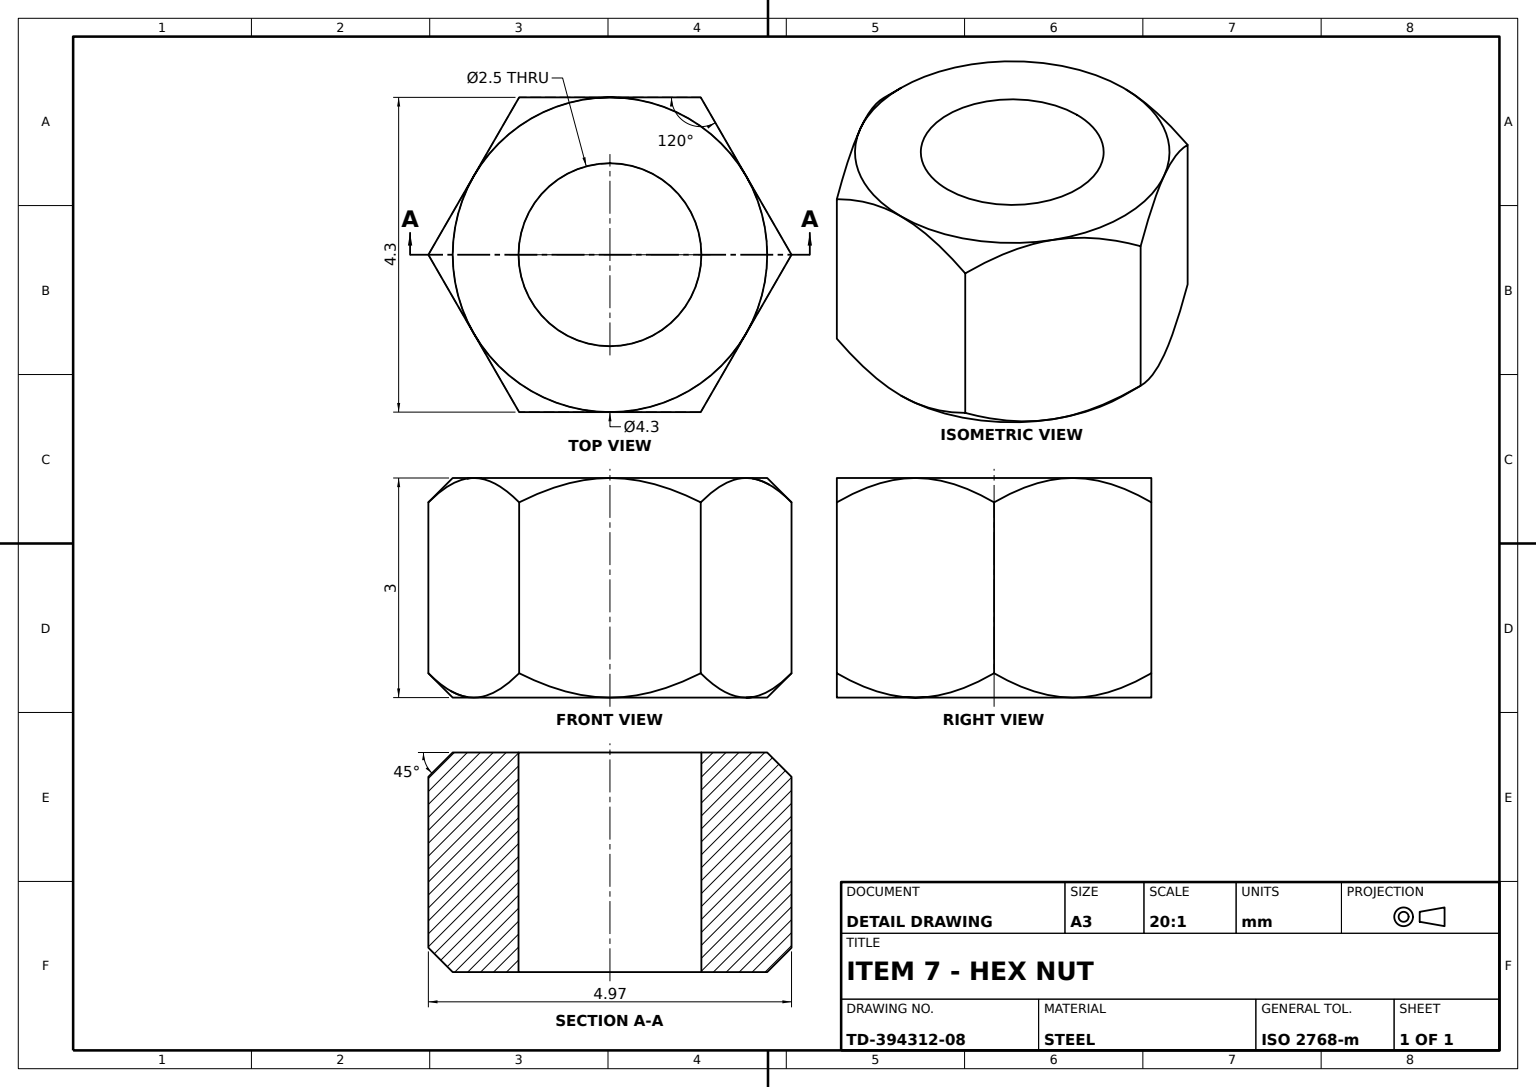
ISO-10303-21;
HEADER;
FILE_DESCRIPTION((''),'2;1');
FILE_NAME('','',(''),(''),'','','');
FILE_SCHEMA(('AUTOMOTIVE_DESIGN'));
ENDSEC;
DATA;
#1=APPLICATION_CONTEXT('');
#2=PRODUCT_CONTEXT('',#1,'mechanical');
#3=PRODUCT('','','',(#2));
#4=PRODUCT_DEFINITION_FORMATION('','',#3);
#5=PRODUCT_DEFINITION_CONTEXT('',#1,'design');
#6=PRODUCT_DEFINITION('','',#4,#5);
#7=PRODUCT_DEFINITION_SHAPE('','',#6);
#8=(LENGTH_UNIT()NAMED_UNIT(*)SI_UNIT(.MILLI.,.METRE.));
#9=(NAMED_UNIT(*)PLANE_ANGLE_UNIT()SI_UNIT($,.RADIAN.));
#10=(NAMED_UNIT(*)SI_UNIT($,.STERADIAN.)SOLID_ANGLE_UNIT());
#11=UNCERTAINTY_MEASURE_WITH_UNIT(LENGTH_MEASURE(1.E-05),#8,'distance_accuracy_value','');
#12=(GEOMETRIC_REPRESENTATION_CONTEXT(3)GLOBAL_UNCERTAINTY_ASSIGNED_CONTEXT((#11))GLOBAL_UNIT_ASSIGNED_CONTEXT((#8,#9,#10))REPRESENTATION_CONTEXT('',''));
#13=CARTESIAN_POINT('',(-1.861955,3.,-1.075));
#14=VERTEX_POINT('',#13);
#15=CARTESIAN_POINT('',(-2.482606,2.667394,0.));
#16=VERTEX_POINT('',#15);
#17=CARTESIAN_POINT('',(-1.969911,3.,-0.888014));
#18=CARTESIAN_POINT('',(-2.076031,2.966986,-0.704208));
#19=CARTESIAN_POINT('',(-2.285328,2.847997,-0.341695));
#20=CARTESIAN_POINT('',(-2.385392,2.764608,-0.16838));
#21=B_SPLINE_CURVE_WITH_KNOTS('',3,(#13,#17,#18,#19,#20,#15),.UNSPECIFIED.,.F.,.F.,(4,2,4),(0.001286977,0.00192583,0.002564683),.UNSPECIFIED.);
#22=EDGE_CURVE('',#14,#16,#21,.T.);
#23=ORIENTED_EDGE('',*,*,#22,.T.);
#24=CARTESIAN_POINT('',(-1.861955,3.,1.075));
#25=VERTEX_POINT('',#24);
#26=CARTESIAN_POINT('',(-2.38528,2.76472,0.168574));
#27=CARTESIAN_POINT('',(-2.28575,2.847423,0.340964));
#28=CARTESIAN_POINT('',(-2.131089,2.935848,0.608845));
#29=CARTESIAN_POINT('',(-2.078631,2.959321,0.699705));
#30=CARTESIAN_POINT('',(-1.971486,2.991467,0.885286));
#31=CARTESIAN_POINT('',(-1.916314,3.,0.980847));
#32=B_SPLINE_CURVE_WITH_KNOTS('',3,(#15,#26,#27,#28,#29,#30,#31,#24),.UNSPECIFIED.,.F.,.F.,(4,2,2,4),(0.000000254,0.000643616,0.000965296,0.001286977),.UNSPECIFIED.);
#33=EDGE_CURVE('',#16,#25,#32,.T.);
#34=ORIENTED_EDGE('',*,*,#33,.T.);
#35=CARTESIAN_POINT('',(0.,3.,0.));
#36=DIRECTION('',(0.,1.,0.));
#37=DIRECTION('',(0.,0.,1.));
#38=AXIS2_PLACEMENT_3D('',#35,#36,#37);
#39=CIRCLE('',#38,2.15);
#40=EDGE_CURVE('',#14,#25,#39,.T.);
#41=ORIENTED_EDGE('',*,*,#40,.F.);
#42=EDGE_LOOP('',(#23,#34,#41));
#43=FACE_OUTER_BOUND('',#42,.T.);
#44=DIRECTION('',(0.,-1.,0.));
#45=AXIS2_PLACEMENT_3D('',#35,#44,#37);
#46=CONICAL_SURFACE('',#45,2.15,0.785398163);
#47=ADVANCED_FACE('',(#43),#46,.T.);
#48=CARTESIAN_POINT('',(0.,0.,-2.15));
#49=VERTEX_POINT('',#48);
#50=CARTESIAN_POINT('',(1.241303,0.332606,-2.15));
#51=VERTEX_POINT('',#50);
#52=CARTESIAN_POINT('',(0.108245,0.,-2.15));
#53=CARTESIAN_POINT('',(0.217598,0.008403,-2.15));
#54=CARTESIAN_POINT('',(0.431131,0.040258,-2.15));
#55=CARTESIAN_POINT('',(0.536253,0.063635,-2.15));
#56=CARTESIAN_POINT('',(0.847499,0.152434,-2.15));
#57=CARTESIAN_POINT('',(1.049442,0.236676,-2.15));
#58=B_SPLINE_CURVE_WITH_KNOTS('',3,(#48,#52,#53,#54,#55,#56,#57,#50),.UNSPECIFIED.,.F.,.F.,(4,2,2,4),(0.005941609,0.00626575,0.006589892,0.007238175),.UNSPECIFIED.);
#59=EDGE_CURVE('',#49,#51,#58,.T.);
#60=ORIENTED_EDGE('',*,*,#59,.F.);
#61=CARTESIAN_POINT('',(-1.241303,0.332606,-2.15));
#62=VERTEX_POINT('',#61);
#63=CARTESIAN_POINT('',(-1.048003,0.235956,-2.15));
#64=CARTESIAN_POINT('',(-0.848605,0.152667,-2.15));
#65=CARTESIAN_POINT('',(-0.429462,0.03325,-2.15));
#66=CARTESIAN_POINT('',(-0.216722,0.,-2.15));
#67=B_SPLINE_CURVE_WITH_KNOTS('',3,(#61,#63,#64,#65,#66,#48),.UNSPECIFIED.,.F.,.F.,(4,2,4),(0.004643657,0.005292633,0.005941609),.UNSPECIFIED.);
#68=EDGE_CURVE('',#62,#49,#67,.T.);
#69=ORIENTED_EDGE('',*,*,#68,.F.);
#70=CARTESIAN_POINT('',(-1.241303,2.667394,-2.15));
#71=VERTEX_POINT('',#70);
#72=CARTESIAN_POINT('',(-1.241303,3.,-2.15));
#73=VECTOR('',#44,1000.);
#74=LINE('',#72,#73);
#75=EDGE_CURVE('',#71,#62,#74,.T.);
#76=ORIENTED_EDGE('',*,*,#75,.F.);
#77=CARTESIAN_POINT('',(0.,3.,-2.15));
#78=VERTEX_POINT('',#77);
#79=CARTESIAN_POINT('',(-0.108083,3.,-2.15));
#80=CARTESIAN_POINT('',(-0.217492,2.991611,-2.15));
#81=CARTESIAN_POINT('',(-0.431167,2.959739,-2.15));
#82=CARTESIAN_POINT('',(-0.536296,2.936353,-2.15));
#83=CARTESIAN_POINT('',(-0.847415,2.84759,-2.15));
#84=CARTESIAN_POINT('',(-1.049403,2.763344,-2.15));
#85=B_SPLINE_CURVE_WITH_KNOTS('',3,(#77,#79,#80,#81,#82,#83,#84,#70),.UNSPECIFIED.,.F.,.F.,(4,2,2,4),(0.005856882,0.006180911,0.006504941,0.007153001),.UNSPECIFIED.);
#86=EDGE_CURVE('',#78,#71,#85,.T.);
#87=ORIENTED_EDGE('',*,*,#86,.F.);
#88=CARTESIAN_POINT('',(1.241303,2.667394,-2.15));
#89=VERTEX_POINT('',#88);
#90=CARTESIAN_POINT('',(1.047934,2.764079,-2.15));
#91=CARTESIAN_POINT('',(0.848699,2.84729,-2.15));
#92=CARTESIAN_POINT('',(0.429757,2.966682,-2.15));
#93=CARTESIAN_POINT('',(0.216465,3.,-2.15));
#94=B_SPLINE_CURVE_WITH_KNOTS('',3,(#88,#90,#91,#92,#93,#77),.UNSPECIFIED.,.F.,.F.,(4,2,4),(0.004558973,0.005207927,0.005856882),.UNSPECIFIED.);
#95=EDGE_CURVE('',#89,#78,#94,.T.);
#96=ORIENTED_EDGE('',*,*,#95,.F.);
#97=CARTESIAN_POINT('',(1.241303,3.,-2.15));
#98=LINE('',#97,#73);
#99=EDGE_CURVE('',#89,#51,#98,.T.);
#100=ORIENTED_EDGE('',*,*,#99,.T.);
#101=EDGE_LOOP('',(#60,#69,#76,#87,#96,#100));
#102=FACE_OUTER_BOUND('',#101,.T.);
#103=DIRECTION('',(1.,0.,0.));
#104=AXIS2_PLACEMENT_3D('',#97,#37,#103);
#105=PLANE('',#104);
#106=ADVANCED_FACE('',(#102),#105,.F.);
#107=ORIENTED_EDGE('',*,*,#99,.F.);
#108=CARTESIAN_POINT('',(1.861955,3.,-1.075));
#109=VERTEX_POINT('',#108);
#110=CARTESIAN_POINT('',(1.753998,3.,-1.261986));
#111=CARTESIAN_POINT('',(1.647878,2.966986,-1.445792));
#112=CARTESIAN_POINT('',(1.438581,2.847997,-1.808305));
#113=CARTESIAN_POINT('',(1.338517,2.764608,-1.98162));
#114=B_SPLINE_CURVE_WITH_KNOTS('',3,(#108,#110,#111,#112,#113,#88),.UNSPECIFIED.,.F.,.F.,(4,2,4),(0.001286977,0.00192583,0.002564683),.UNSPECIFIED.);
#115=EDGE_CURVE('',#109,#89,#114,.T.);
#116=ORIENTED_EDGE('',*,*,#115,.F.);
#117=CARTESIAN_POINT('',(2.482606,2.667394,0.));
#118=VERTEX_POINT('',#117);
#119=CARTESIAN_POINT('',(2.38528,2.76472,-0.168574));
#120=CARTESIAN_POINT('',(2.28575,2.847423,-0.340964));
#121=CARTESIAN_POINT('',(2.131089,2.935848,-0.608845));
#122=CARTESIAN_POINT('',(2.078631,2.959321,-0.699705));
#123=CARTESIAN_POINT('',(1.971486,2.991467,-0.885286));
#124=CARTESIAN_POINT('',(1.916314,3.,-0.980847));
#125=B_SPLINE_CURVE_WITH_KNOTS('',3,(#117,#119,#120,#121,#122,#123,#124,#108),.UNSPECIFIED.,.F.,.F.,(4,2,2,4),(0.000000254,0.000643616,0.000965296,0.001286977),.UNSPECIFIED.);
#126=EDGE_CURVE('',#118,#109,#125,.T.);
#127=ORIENTED_EDGE('',*,*,#126,.F.);
#128=CARTESIAN_POINT('',(2.482606,0.332606,0.));
#129=VERTEX_POINT('',#128);
#130=CARTESIAN_POINT('',(2.482606,3.,0.));
#131=LINE('',#130,#73);
#132=EDGE_CURVE('',#118,#129,#131,.T.);
#133=ORIENTED_EDGE('',*,*,#132,.T.);
#134=CARTESIAN_POINT('',(1.861955,0.,-1.075));
#135=VERTEX_POINT('',#134);
#136=CARTESIAN_POINT('',(1.969911,0.,-0.888014));
#137=CARTESIAN_POINT('',(2.076031,0.033014,-0.704208));
#138=CARTESIAN_POINT('',(2.285328,0.152003,-0.341695));
#139=CARTESIAN_POINT('',(2.385392,0.235392,-0.16838));
#140=B_SPLINE_CURVE_WITH_KNOTS('',3,(#134,#136,#137,#138,#139,#128),.UNSPECIFIED.,.F.,.F.,(4,2,4),(0.001286977,0.00192583,0.002564683),.UNSPECIFIED.);
#141=EDGE_CURVE('',#135,#129,#140,.T.);
#142=ORIENTED_EDGE('',*,*,#141,.F.);
#143=CARTESIAN_POINT('',(1.33863,0.23528,-1.981426));
#144=CARTESIAN_POINT('',(1.438159,0.152577,-1.809036));
#145=CARTESIAN_POINT('',(1.59282,0.064152,-1.541155));
#146=CARTESIAN_POINT('',(1.645278,0.040679,-1.450295));
#147=CARTESIAN_POINT('',(1.752423,0.008533,-1.264714));
#148=CARTESIAN_POINT('',(1.807596,0.,-1.169153));
#149=B_SPLINE_CURVE_WITH_KNOTS('',3,(#50,#143,#144,#145,#146,#147,#148,#134),.UNSPECIFIED.,.F.,.F.,(4,2,2,4),(0.000000254,0.000643616,0.000965296,0.001286977),.UNSPECIFIED.);
#150=EDGE_CURVE('',#51,#135,#149,.T.);
#151=ORIENTED_EDGE('',*,*,#150,.F.);
#152=EDGE_LOOP('',(#107,#116,#127,#133,#142,#151));
#153=FACE_OUTER_BOUND('',#152,.T.);
#154=DIRECTION('',(-0.866025404,0.,0.5));
#155=DIRECTION('',(0.5,0.,0.866025404));
#156=AXIS2_PLACEMENT_3D('',#130,#154,#155);
#157=PLANE('',#156);
#158=ADVANCED_FACE('',(#153),#157,.F.);
#159=CARTESIAN_POINT('',(0.,3.,-1.25));
#160=VERTEX_POINT('',#159);
#161=CARTESIAN_POINT('',(0.,0.,-1.25));
#162=VERTEX_POINT('',#161);
#163=CARTESIAN_POINT('',(0.,23.,-1.25));
#164=LINE('',#163,#73);
#165=EDGE_CURVE('',#160,#162,#164,.T.);
#166=ORIENTED_EDGE('',*,*,#165,.T.);
#167=CARTESIAN_POINT('',(0.,0.,1.25));
#168=VERTEX_POINT('',#167);
#169=CARTESIAN_POINT('',(0.,0.,0.));
#170=DIRECTION('',(0.,0.,-1.));
#171=AXIS2_PLACEMENT_3D('',#169,#44,#170);
#172=CIRCLE('',#171,1.25);
#173=EDGE_CURVE('',#162,#168,#172,.T.);
#174=ORIENTED_EDGE('',*,*,#173,.T.);
#175=CARTESIAN_POINT('',(0.,3.,1.25));
#176=VERTEX_POINT('',#175);
#177=CARTESIAN_POINT('',(0.,23.,1.25));
#178=LINE('',#177,#73);
#179=EDGE_CURVE('',#176,#168,#178,.T.);
#180=ORIENTED_EDGE('',*,*,#179,.F.);
#181=CIRCLE('',#38,1.25);
#182=EDGE_CURVE('',#176,#160,#181,.T.);
#183=ORIENTED_EDGE('',*,*,#182,.T.);
#184=EDGE_LOOP('',(#166,#174,#180,#183));
#185=FACE_OUTER_BOUND('',#184,.T.);
#186=CARTESIAN_POINT('',(0.,23.,0.));
#187=AXIS2_PLACEMENT_3D('',#186,#44,#170);
#188=CYLINDRICAL_SURFACE('',#187,1.25);
#189=ADVANCED_FACE('',(#185),#188,.F.);
#190=CARTESIAN_POINT('',(1.241303,2.667394,2.15));
#191=VERTEX_POINT('',#190);
#192=CARTESIAN_POINT('',(1.861955,3.,1.075));
#193=VERTEX_POINT('',#192);
#194=CARTESIAN_POINT('',(1.33863,2.76472,1.981426));
#195=CARTESIAN_POINT('',(1.438159,2.847423,1.809036));
#196=CARTESIAN_POINT('',(1.59282,2.935848,1.541155));
#197=CARTESIAN_POINT('',(1.645278,2.959321,1.450295));
#198=CARTESIAN_POINT('',(1.752423,2.991467,1.264714));
#199=CARTESIAN_POINT('',(1.807596,3.,1.169153));
#200=B_SPLINE_CURVE_WITH_KNOTS('',3,(#190,#194,#195,#196,#197,#198,#199,#192),.UNSPECIFIED.,.F.,.F.,(4,2,2,4),(0.000000254,0.000643616,0.000965296,0.001286977),.UNSPECIFIED.);
#201=EDGE_CURVE('',#191,#193,#200,.T.);
#202=ORIENTED_EDGE('',*,*,#201,.T.);
#203=CARTESIAN_POINT('',(0.,3.,2.15));
#204=VERTEX_POINT('',#203);
#205=EDGE_CURVE('',#204,#193,#39,.T.);
#206=ORIENTED_EDGE('',*,*,#205,.F.);
#207=CARTESIAN_POINT('',(0.108083,3.,2.15));
#208=CARTESIAN_POINT('',(0.217492,2.991611,2.15));
#209=CARTESIAN_POINT('',(0.431167,2.959739,2.15));
#210=CARTESIAN_POINT('',(0.536296,2.936353,2.15));
#211=CARTESIAN_POINT('',(0.847415,2.84759,2.15));
#212=CARTESIAN_POINT('',(1.049403,2.763344,2.15));
#213=B_SPLINE_CURVE_WITH_KNOTS('',3,(#203,#207,#208,#209,#210,#211,#212,#190),.UNSPECIFIED.,.F.,.F.,(4,2,2,4),(0.005856882,0.006180911,0.006504941,0.007153001),.UNSPECIFIED.);
#214=EDGE_CURVE('',#204,#191,#213,.T.);
#215=ORIENTED_EDGE('',*,*,#214,.T.);
#216=EDGE_LOOP('',(#202,#206,#215));
#217=FACE_OUTER_BOUND('',#216,.T.);
#218=ADVANCED_FACE('',(#217),#46,.T.);
#219=EDGE_CURVE('',#78,#14,#39,.T.);
#220=ORIENTED_EDGE('',*,*,#219,.F.);
#221=ORIENTED_EDGE('',*,*,#86,.T.);
#222=CARTESIAN_POINT('',(-1.33863,2.76472,-1.981426));
#223=CARTESIAN_POINT('',(-1.438159,2.847423,-1.809036));
#224=CARTESIAN_POINT('',(-1.59282,2.935848,-1.541155));
#225=CARTESIAN_POINT('',(-1.645278,2.959321,-1.450295));
#226=CARTESIAN_POINT('',(-1.752423,2.991467,-1.264714));
#227=CARTESIAN_POINT('',(-1.807596,3.,-1.169153));
#228=B_SPLINE_CURVE_WITH_KNOTS('',3,(#70,#222,#223,#224,#225,#226,#227,#13),.UNSPECIFIED.,.F.,.F.,(4,2,2,4),(0.000000254,0.000643616,0.000965296,0.001286977),.UNSPECIFIED.);
#229=EDGE_CURVE('',#71,#14,#228,.T.);
#230=ORIENTED_EDGE('',*,*,#229,.T.);
#231=EDGE_LOOP('',(#220,#221,#230));
#232=FACE_OUTER_BOUND('',#231,.T.);
#233=ADVANCED_FACE('',(#232),#46,.T.);
#234=CARTESIAN_POINT('',(-1.241303,2.667394,2.15));
#235=VERTEX_POINT('',#234);
#236=CARTESIAN_POINT('',(-1.753998,3.,1.261986));
#237=CARTESIAN_POINT('',(-1.647878,2.966986,1.445792));
#238=CARTESIAN_POINT('',(-1.438581,2.847997,1.808305));
#239=CARTESIAN_POINT('',(-1.338517,2.764608,1.98162));
#240=B_SPLINE_CURVE_WITH_KNOTS('',3,(#24,#236,#237,#238,#239,#234),.UNSPECIFIED.,.F.,.F.,(4,2,4),(0.001286977,0.00192583,0.002564683),.UNSPECIFIED.);
#241=EDGE_CURVE('',#25,#235,#240,.T.);
#242=ORIENTED_EDGE('',*,*,#241,.T.);
#243=CARTESIAN_POINT('',(-1.047934,2.764079,2.15));
#244=CARTESIAN_POINT('',(-0.848699,2.84729,2.15));
#245=CARTESIAN_POINT('',(-0.429757,2.966682,2.15));
#246=CARTESIAN_POINT('',(-0.216465,3.,2.15));
#247=B_SPLINE_CURVE_WITH_KNOTS('',3,(#234,#243,#244,#245,#246,#203),.UNSPECIFIED.,.F.,.F.,(4,2,4),(0.004558973,0.005207927,0.005856882),.UNSPECIFIED.);
#248=EDGE_CURVE('',#235,#204,#247,.T.);
#249=ORIENTED_EDGE('',*,*,#248,.T.);
#250=EDGE_CURVE('',#25,#204,#39,.T.);
#251=ORIENTED_EDGE('',*,*,#250,.F.);
#252=EDGE_LOOP('',(#242,#249,#251));
#253=FACE_OUTER_BOUND('',#252,.T.);
#254=ADVANCED_FACE('',(#253),#46,.T.);
#255=CARTESIAN_POINT('',(-2.482606,0.332606,0.));
#256=VERTEX_POINT('',#255);
#257=CARTESIAN_POINT('',(-1.861955,0.,-1.075));
#258=VERTEX_POINT('',#257);
#259=CARTESIAN_POINT('',(-2.38528,0.23528,-0.168574));
#260=CARTESIAN_POINT('',(-2.28575,0.152577,-0.340964));
#261=CARTESIAN_POINT('',(-2.131089,0.064152,-0.608845));
#262=CARTESIAN_POINT('',(-2.078631,0.040679,-0.699705));
#263=CARTESIAN_POINT('',(-1.971486,0.008533,-0.885286));
#264=CARTESIAN_POINT('',(-1.916314,0.,-0.980847));
#265=B_SPLINE_CURVE_WITH_KNOTS('',3,(#255,#259,#260,#261,#262,#263,#264,#257),.UNSPECIFIED.,.F.,.F.,(4,2,2,4),(0.000000254,0.000643616,0.000965296,0.001286977),.UNSPECIFIED.);
#266=EDGE_CURVE('',#256,#258,#265,.T.);
#267=ORIENTED_EDGE('',*,*,#266,.T.);
#268=CARTESIAN_POINT('',(-1.861955,0.,1.075));
#269=VERTEX_POINT('',#268);
#270=AXIS2_PLACEMENT_3D('',#169,#36,#37);
#271=CIRCLE('',#270,2.15);
#272=EDGE_CURVE('',#258,#269,#271,.T.);
#273=ORIENTED_EDGE('',*,*,#272,.T.);
#274=CARTESIAN_POINT('',(-1.969911,0.,0.888014));
#275=CARTESIAN_POINT('',(-2.076031,0.033014,0.704208));
#276=CARTESIAN_POINT('',(-2.285328,0.152003,0.341695));
#277=CARTESIAN_POINT('',(-2.385392,0.235392,0.16838));
#278=B_SPLINE_CURVE_WITH_KNOTS('',3,(#268,#274,#275,#276,#277,#255),.UNSPECIFIED.,.F.,.F.,(4,2,4),(0.001286977,0.00192583,0.002564683),.UNSPECIFIED.);
#279=EDGE_CURVE('',#269,#256,#278,.T.);
#280=ORIENTED_EDGE('',*,*,#279,.T.);
#281=EDGE_LOOP('',(#267,#273,#280));
#282=FACE_OUTER_BOUND('',#281,.T.);
#283=AXIS2_PLACEMENT_3D('',#169,#36,#170);
#284=CONICAL_SURFACE('',#283,2.15,0.785398163);
#285=ADVANCED_FACE('',(#282),#284,.T.);
#286=CARTESIAN_POINT('',(1.241303,0.332606,2.15));
#287=VERTEX_POINT('',#286);
#288=CARTESIAN_POINT('',(0.,0.,2.15));
#289=VERTEX_POINT('',#288);
#290=CARTESIAN_POINT('',(1.048003,0.235956,2.15));
#291=CARTESIAN_POINT('',(0.848605,0.152667,2.15));
#292=CARTESIAN_POINT('',(0.429462,0.03325,2.15));
#293=CARTESIAN_POINT('',(0.216722,0.,2.15));
#294=B_SPLINE_CURVE_WITH_KNOTS('',3,(#286,#290,#291,#292,#293,#288),.UNSPECIFIED.,.F.,.F.,(4,2,4),(0.004643657,0.005292633,0.005941609),.UNSPECIFIED.);
#295=EDGE_CURVE('',#287,#289,#294,.T.);
#296=ORIENTED_EDGE('',*,*,#295,.F.);
#297=CARTESIAN_POINT('',(1.241303,3.,2.15));
#298=LINE('',#297,#73);
#299=EDGE_CURVE('',#191,#287,#298,.T.);
#300=ORIENTED_EDGE('',*,*,#299,.F.);
#301=ORIENTED_EDGE('',*,*,#214,.F.);
#302=ORIENTED_EDGE('',*,*,#248,.F.);
#303=CARTESIAN_POINT('',(-1.241303,0.332606,2.15));
#304=VERTEX_POINT('',#303);
#305=CARTESIAN_POINT('',(-1.241303,3.,2.15));
#306=LINE('',#305,#73);
#307=EDGE_CURVE('',#235,#304,#306,.T.);
#308=ORIENTED_EDGE('',*,*,#307,.T.);
#309=CARTESIAN_POINT('',(-0.108245,0.,2.15));
#310=CARTESIAN_POINT('',(-0.217598,0.008403,2.15));
#311=CARTESIAN_POINT('',(-0.431131,0.040258,2.15));
#312=CARTESIAN_POINT('',(-0.536253,0.063635,2.15));
#313=CARTESIAN_POINT('',(-0.847499,0.152434,2.15));
#314=CARTESIAN_POINT('',(-1.049442,0.236676,2.15));
#315=B_SPLINE_CURVE_WITH_KNOTS('',3,(#288,#309,#310,#311,#312,#313,#314,#303),.UNSPECIFIED.,.F.,.F.,(4,2,2,4),(0.005941609,0.00626575,0.006589892,0.007238175),.UNSPECIFIED.);
#316=EDGE_CURVE('',#289,#304,#315,.T.);
#317=ORIENTED_EDGE('',*,*,#316,.F.);
#318=EDGE_LOOP('',(#296,#300,#301,#302,#308,#317));
#319=FACE_OUTER_BOUND('',#318,.T.);
#320=DIRECTION('',(-1.,0.,0.));
#321=AXIS2_PLACEMENT_3D('',#305,#170,#320);
#322=PLANE('',#321);
#323=ADVANCED_FACE('',(#319),#322,.F.);
#324=ORIENTED_EDGE('',*,*,#150,.T.);
#325=CIRCLE('',#171,2.15);
#326=EDGE_CURVE('',#49,#135,#325,.T.);
#327=ORIENTED_EDGE('',*,*,#326,.F.);
#328=ORIENTED_EDGE('',*,*,#59,.T.);
#329=EDGE_LOOP('',(#324,#327,#328));
#330=FACE_OUTER_BOUND('',#329,.T.);
#331=ADVANCED_FACE('',(#330),#284,.T.);
#332=CARTESIAN_POINT('',(1.861955,0.,1.075));
#333=VERTEX_POINT('',#332);
#334=CARTESIAN_POINT('',(1.753998,0.,1.261986));
#335=CARTESIAN_POINT('',(1.647878,0.033014,1.445792));
#336=CARTESIAN_POINT('',(1.438581,0.152003,1.808305));
#337=CARTESIAN_POINT('',(1.338517,0.235392,1.98162));
#338=B_SPLINE_CURVE_WITH_KNOTS('',3,(#332,#334,#335,#336,#337,#286),.UNSPECIFIED.,.F.,.F.,(4,2,4),(0.001286977,0.00192583,0.002564683),.UNSPECIFIED.);
#339=EDGE_CURVE('',#333,#287,#338,.T.);
#340=ORIENTED_EDGE('',*,*,#339,.F.);
#341=CARTESIAN_POINT('',(2.38528,0.23528,0.168574));
#342=CARTESIAN_POINT('',(2.28575,0.152577,0.340964));
#343=CARTESIAN_POINT('',(2.131089,0.064152,0.608845));
#344=CARTESIAN_POINT('',(2.078631,0.040679,0.699705));
#345=CARTESIAN_POINT('',(1.971486,0.008533,0.885286));
#346=CARTESIAN_POINT('',(1.916314,0.,0.980847));
#347=B_SPLINE_CURVE_WITH_KNOTS('',3,(#128,#341,#342,#343,#344,#345,#346,#332),.UNSPECIFIED.,.F.,.F.,(4,2,2,4),(0.000000254,0.000643616,0.000965296,0.001286977),.UNSPECIFIED.);
#348=EDGE_CURVE('',#129,#333,#347,.T.);
#349=ORIENTED_EDGE('',*,*,#348,.F.);
#350=ORIENTED_EDGE('',*,*,#132,.F.);
#351=CARTESIAN_POINT('',(1.969911,3.,0.888014));
#352=CARTESIAN_POINT('',(2.076031,2.966986,0.704208));
#353=CARTESIAN_POINT('',(2.285328,2.847997,0.341695));
#354=CARTESIAN_POINT('',(2.385392,2.764608,0.16838));
#355=B_SPLINE_CURVE_WITH_KNOTS('',3,(#192,#351,#352,#353,#354,#117),.UNSPECIFIED.,.F.,.F.,(4,2,4),(0.001286977,0.00192583,0.002564683),.UNSPECIFIED.);
#356=EDGE_CURVE('',#193,#118,#355,.T.);
#357=ORIENTED_EDGE('',*,*,#356,.F.);
#358=ORIENTED_EDGE('',*,*,#201,.F.);
#359=ORIENTED_EDGE('',*,*,#299,.T.);
#360=EDGE_LOOP('',(#340,#349,#350,#357,#358,#359));
#361=FACE_OUTER_BOUND('',#360,.T.);
#362=DIRECTION('',(-0.866025404,0.,-0.5));
#363=DIRECTION('',(-0.5,0.,0.866025404));
#364=AXIS2_PLACEMENT_3D('',#297,#362,#363);
#365=PLANE('',#364);
#366=ADVANCED_FACE('',(#361),#365,.F.);
#367=EDGE_CURVE('',#168,#162,#172,.T.);
#368=ORIENTED_EDGE('',*,*,#367,.F.);
#369=ORIENTED_EDGE('',*,*,#173,.F.);
#370=EDGE_LOOP('',(#368,#369));
#371=FACE_BOUND('',#370,.T.);
#372=EDGE_CURVE('',#289,#333,#271,.T.);
#373=ORIENTED_EDGE('',*,*,#372,.F.);
#374=EDGE_CURVE('',#269,#289,#271,.T.);
#375=ORIENTED_EDGE('',*,*,#374,.F.);
#376=ORIENTED_EDGE('',*,*,#272,.F.);
#377=EDGE_CURVE('',#49,#258,#271,.T.);
#378=ORIENTED_EDGE('',*,*,#377,.F.);
#379=ORIENTED_EDGE('',*,*,#326,.T.);
#380=EDGE_CURVE('',#333,#135,#271,.T.);
#381=ORIENTED_EDGE('',*,*,#380,.F.);
#382=EDGE_LOOP('',(#373,#375,#376,#378,#379,#381));
#383=FACE_OUTER_BOUND('',#382,.T.);
#384=PLANE('',#270);
#385=ADVANCED_FACE('',(#371,#383),#384,.F.);
#386=ORIENTED_EDGE('',*,*,#179,.T.);
#387=ORIENTED_EDGE('',*,*,#367,.T.);
#388=ORIENTED_EDGE('',*,*,#165,.F.);
#389=EDGE_CURVE('',#160,#176,#181,.T.);
#390=ORIENTED_EDGE('',*,*,#389,.T.);
#391=EDGE_LOOP('',(#386,#387,#388,#390));
#392=FACE_OUTER_BOUND('',#391,.T.);
#393=ADVANCED_FACE('',(#392),#188,.F.);
#394=ORIENTED_EDGE('',*,*,#95,.T.);
#395=EDGE_CURVE('',#109,#78,#39,.T.);
#396=ORIENTED_EDGE('',*,*,#395,.F.);
#397=ORIENTED_EDGE('',*,*,#115,.T.);
#398=EDGE_LOOP('',(#394,#396,#397));
#399=FACE_OUTER_BOUND('',#398,.T.);
#400=ADVANCED_FACE('',(#399),#46,.T.);
#401=CARTESIAN_POINT('',(-1.33863,0.23528,1.981426));
#402=CARTESIAN_POINT('',(-1.438159,0.152577,1.809036));
#403=CARTESIAN_POINT('',(-1.59282,0.064152,1.541155));
#404=CARTESIAN_POINT('',(-1.645278,0.040679,1.450295));
#405=CARTESIAN_POINT('',(-1.752423,0.008533,1.264714));
#406=CARTESIAN_POINT('',(-1.807596,0.,1.169153));
#407=B_SPLINE_CURVE_WITH_KNOTS('',3,(#303,#401,#402,#403,#404,#405,#406,#268),.UNSPECIFIED.,.F.,.F.,(4,2,2,4),(0.000000254,0.000643616,0.000965296,0.001286977),.UNSPECIFIED.);
#408=EDGE_CURVE('',#304,#269,#407,.T.);
#409=ORIENTED_EDGE('',*,*,#408,.T.);
#410=ORIENTED_EDGE('',*,*,#374,.T.);
#411=ORIENTED_EDGE('',*,*,#316,.T.);
#412=EDGE_LOOP('',(#409,#410,#411));
#413=FACE_OUTER_BOUND('',#412,.T.);
#414=ADVANCED_FACE('',(#413),#284,.T.);
#415=ORIENTED_EDGE('',*,*,#389,.F.);
#416=ORIENTED_EDGE('',*,*,#182,.F.);
#417=EDGE_LOOP('',(#415,#416));
#418=FACE_BOUND('',#417,.T.);
#419=ORIENTED_EDGE('',*,*,#250,.T.);
#420=ORIENTED_EDGE('',*,*,#205,.T.);
#421=EDGE_CURVE('',#193,#109,#39,.T.);
#422=ORIENTED_EDGE('',*,*,#421,.T.);
#423=ORIENTED_EDGE('',*,*,#395,.T.);
#424=ORIENTED_EDGE('',*,*,#219,.T.);
#425=ORIENTED_EDGE('',*,*,#40,.T.);
#426=EDGE_LOOP('',(#419,#420,#422,#423,#424,#425));
#427=FACE_OUTER_BOUND('',#426,.T.);
#428=PLANE('',#38);
#429=ADVANCED_FACE('',(#418,#427),#428,.T.);
#430=ORIENTED_EDGE('',*,*,#68,.T.);
#431=ORIENTED_EDGE('',*,*,#377,.T.);
#432=CARTESIAN_POINT('',(-1.753998,0.,-1.261986));
#433=CARTESIAN_POINT('',(-1.647878,0.033014,-1.445792));
#434=CARTESIAN_POINT('',(-1.438581,0.152003,-1.808305));
#435=CARTESIAN_POINT('',(-1.338517,0.235392,-1.98162));
#436=B_SPLINE_CURVE_WITH_KNOTS('',3,(#257,#432,#433,#434,#435,#61),.UNSPECIFIED.,.F.,.F.,(4,2,4),(0.001286977,0.00192583,0.002564683),.UNSPECIFIED.);
#437=EDGE_CURVE('',#258,#62,#436,.T.);
#438=ORIENTED_EDGE('',*,*,#437,.T.);
#439=EDGE_LOOP('',(#430,#431,#438));
#440=FACE_OUTER_BOUND('',#439,.T.);
#441=ADVANCED_FACE('',(#440),#284,.T.);
#442=ORIENTED_EDGE('',*,*,#437,.F.);
#443=ORIENTED_EDGE('',*,*,#266,.F.);
#444=CARTESIAN_POINT('',(-2.482606,3.,0.));
#445=LINE('',#444,#73);
#446=EDGE_CURVE('',#16,#256,#445,.T.);
#447=ORIENTED_EDGE('',*,*,#446,.F.);
#448=ORIENTED_EDGE('',*,*,#22,.F.);
#449=ORIENTED_EDGE('',*,*,#229,.F.);
#450=ORIENTED_EDGE('',*,*,#75,.T.);
#451=EDGE_LOOP('',(#442,#443,#447,#448,#449,#450));
#452=FACE_OUTER_BOUND('',#451,.T.);
#453=DIRECTION('',(0.866025404,0.,0.5));
#454=DIRECTION('',(0.5,0.,-0.866025404));
#455=AXIS2_PLACEMENT_3D('',#72,#453,#454);
#456=PLANE('',#455);
#457=ADVANCED_FACE('',(#452),#456,.F.);
#458=ORIENTED_EDGE('',*,*,#348,.T.);
#459=ORIENTED_EDGE('',*,*,#380,.T.);
#460=ORIENTED_EDGE('',*,*,#141,.T.);
#461=EDGE_LOOP('',(#458,#459,#460));
#462=FACE_OUTER_BOUND('',#461,.T.);
#463=ADVANCED_FACE('',(#462),#284,.T.);
#464=ORIENTED_EDGE('',*,*,#307,.F.);
#465=ORIENTED_EDGE('',*,*,#241,.F.);
#466=ORIENTED_EDGE('',*,*,#33,.F.);
#467=ORIENTED_EDGE('',*,*,#446,.T.);
#468=ORIENTED_EDGE('',*,*,#279,.F.);
#469=ORIENTED_EDGE('',*,*,#408,.F.);
#470=EDGE_LOOP('',(#464,#465,#466,#467,#468,#469));
#471=FACE_OUTER_BOUND('',#470,.T.);
#472=DIRECTION('',(0.866025404,0.,-0.5));
#473=DIRECTION('',(-0.5,0.,-0.866025404));
#474=AXIS2_PLACEMENT_3D('',#444,#472,#473);
#475=PLANE('',#474);
#476=ADVANCED_FACE('',(#471),#475,.F.);
#477=ORIENTED_EDGE('',*,*,#339,.T.);
#478=ORIENTED_EDGE('',*,*,#295,.T.);
#479=ORIENTED_EDGE('',*,*,#372,.T.);
#480=EDGE_LOOP('',(#477,#478,#479));
#481=FACE_OUTER_BOUND('',#480,.T.);
#482=ADVANCED_FACE('',(#481),#284,.T.);
#483=ORIENTED_EDGE('',*,*,#126,.T.);
#484=ORIENTED_EDGE('',*,*,#421,.F.);
#485=ORIENTED_EDGE('',*,*,#356,.T.);
#486=EDGE_LOOP('',(#483,#484,#485));
#487=FACE_OUTER_BOUND('',#486,.T.);
#488=ADVANCED_FACE('',(#487),#46,.T.);
#489=CLOSED_SHELL('',(#47,#106,#158,#189,#218,#233,#254,#285,#323,#331,#366,#385,#393,#400,#414,#429,#441,#457,#463,#476,#482,#488));
#490=MANIFOLD_SOLID_BREP('',#489);
#491=ADVANCED_BREP_SHAPE_REPRESENTATION('',(#490),#12);
#492=SHAPE_DEFINITION_REPRESENTATION(#7,#491);
ENDSEC;
END-ISO-10303-21;
